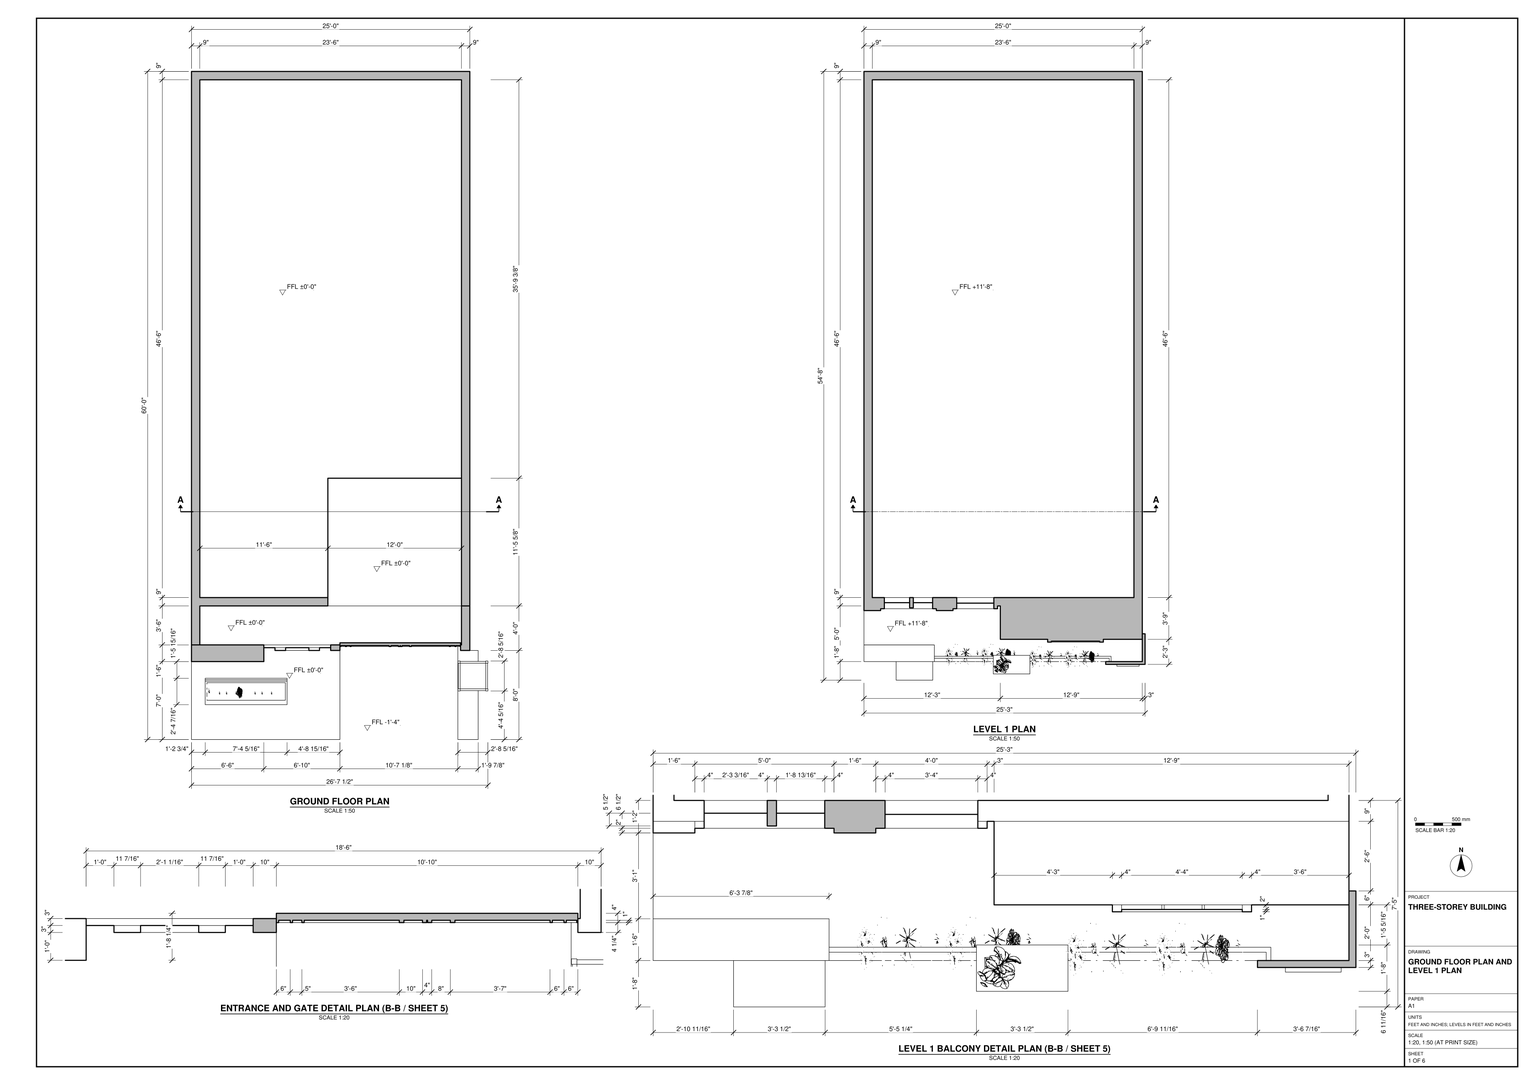
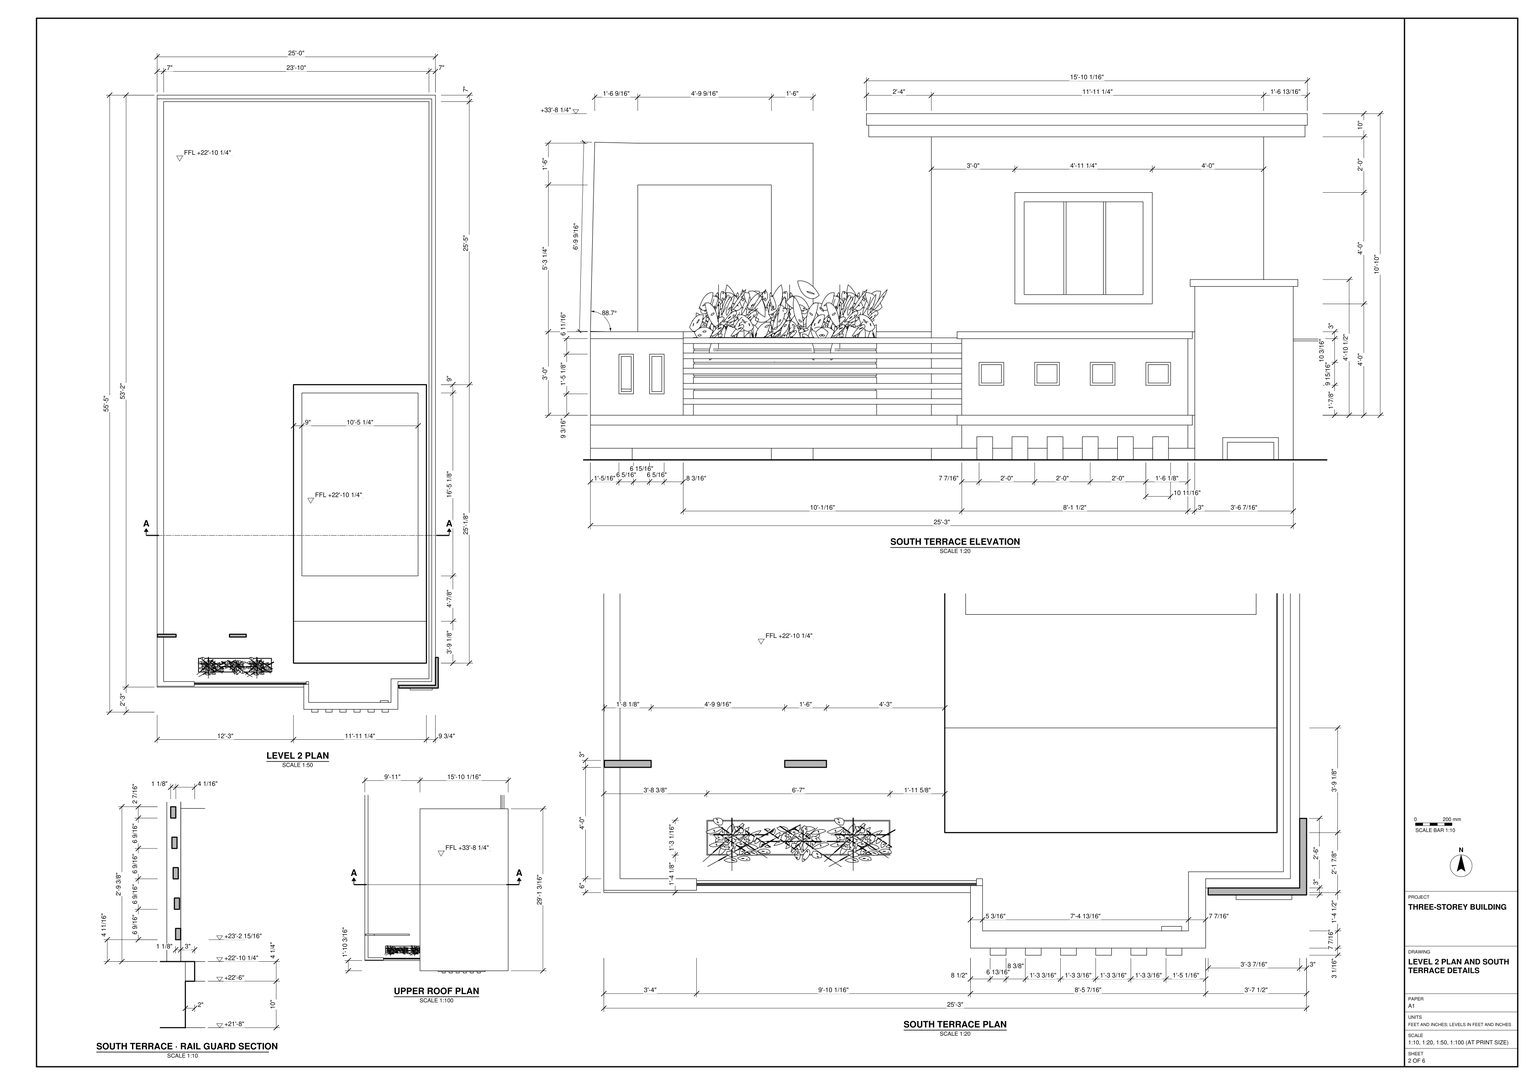
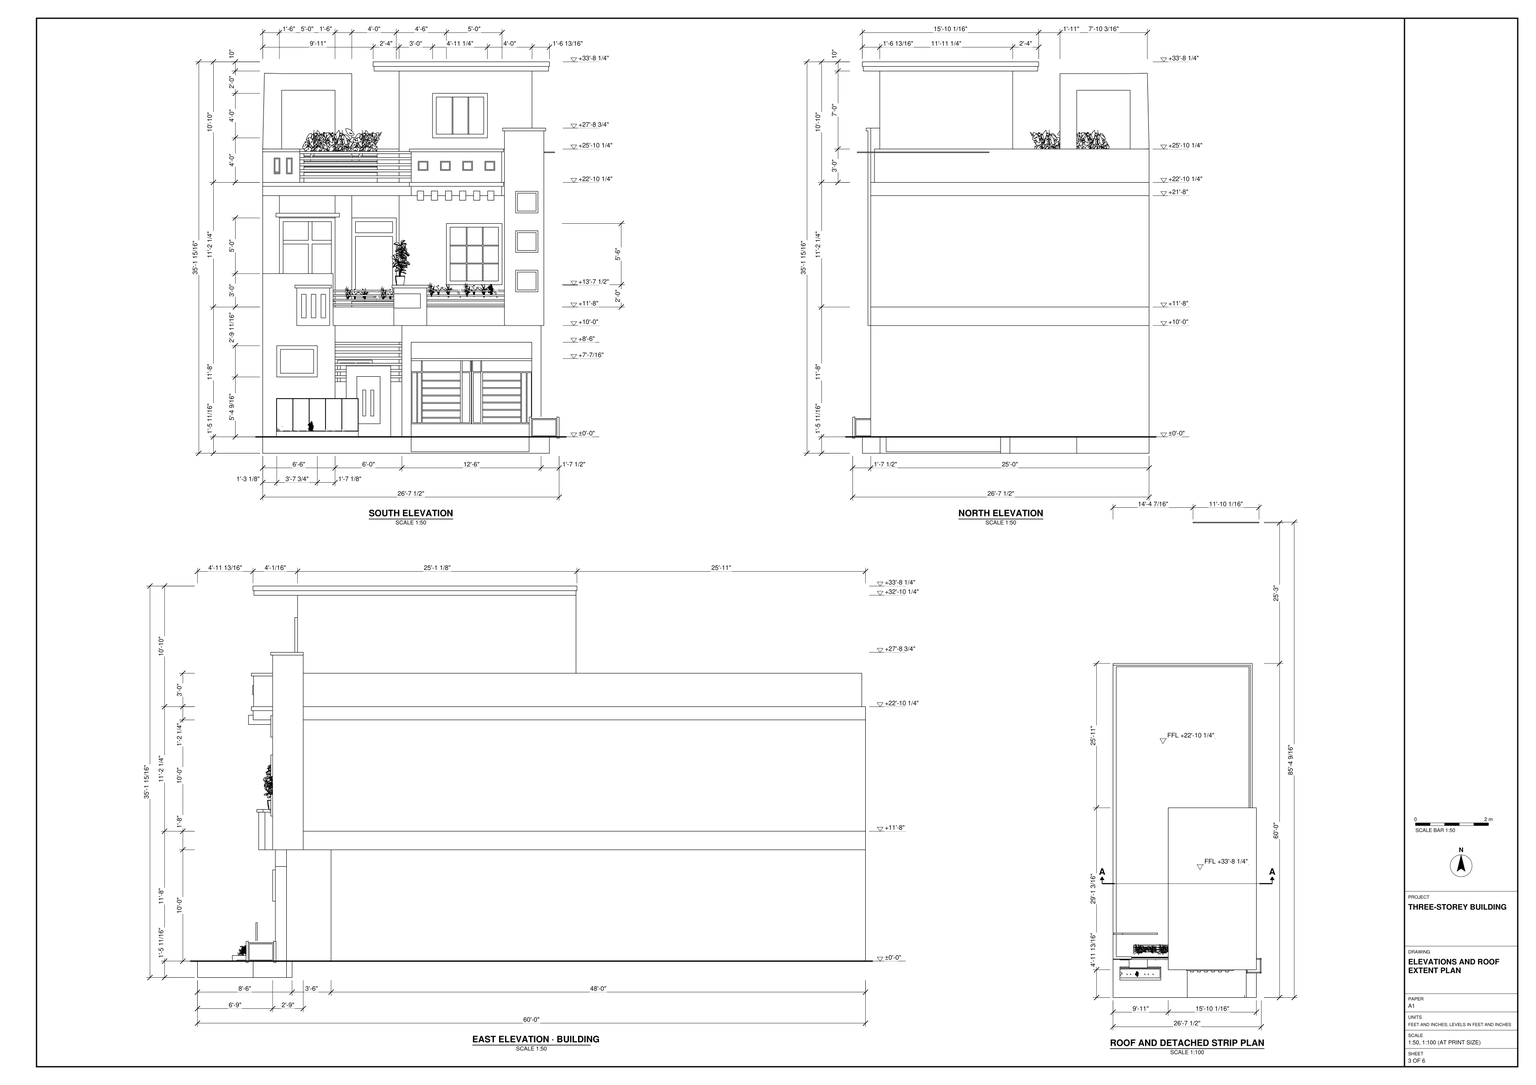
Build the three-storey building in SketchUp from task_files/diagram_01.pdf. Work in feet and inches. The complete model is 26'-7 1/2" wide, 85'-4 9/16" deep and 35'-1 15/16" high. Use finished floor levels of ±0'-0", +11'-8" and +22'-10 1/4". The overall depth includes the detached strip; position it from the roof and detached strip plan rather than extending the building to fill that depth.

Lay out the slabs and walls from the floor plans, using the 9" main perimeter walls on the lower floors and the 7" terrace perimeter walls where dimensioned. Keep the rear and long side elevations plain as drawn. On the south front, model the change in ground level, pedestrian entrance, wider slatted gate and projecting balcony. Set the balcony door and divided windows behind the guard, and carry the tall panelled feature up the right edge of the facade. At terrace level, distinguish the open frame from the roofed enclosure. Follow the terrace details for the parapet openings, horizontal rails and planting positions.

Decor and loose items, including plants, may be any suitable library components, for example from 3D Warehouse. Keep shell elements such as walls, slabs and roofs, and each furniture or joinery piece shown, in separate groups or components. Use components for repeated parts. Save one SketchUp model as output_files/three_storey_building_south_balcony_and_roof_terrace.skp.

# SketchUp Ruby script. Lengths in inches.
U = 1.inch
M = Sketchup.active_model
def pt(a) = Geom::Point3d.new(a.map { |v| v * U })
def face(e, loops, mat)
  f = e.add_face(loops[0].map { |a| pt(a) })
  loops[1..].each { |l| e.add_face(l.map { |a| pt(a) }).erase! }
  f.material = f.back_material = mat if mat
  f
end
# faces: each face lists its corners as indices into pts; further lists are holes
def faces(e, pts, list, mat = nil) = list.each { |f| face(e, (f[0].is_a?(Array) ? f : [f]).map { |l| l.map { |i| pts[i] } }, mat) }
# xy, xz, yz: faces in a plane at the given z, y or x. An outline is a flat list of corners, or four numbers for a rectangle; further outlines are holes
def ring(l) = l.size == 4 ? [[l[0], l[1]], [l[2], l[1]], [l[2], l[3]], [l[0], l[3]]] : l.each_slice(2).to_a
def flat(e, list, mat, &to3) = list.each { |f| face(e, (f[0].is_a?(Array) ? f : [f]).map { |l| ring(l).map { |u, v| to3.(u, v) } }, mat) }
def xy(e, z, list, mat = nil) = flat(e, list, mat) { |x, y| [x, y, z] }
def xz(e, y, list, mat = nil) = flat(e, list, mat) { |x, z| [x, y, z] }
def yz(e, x, list, mat = nil) = flat(e, list, mat) { |y, z| [x, y, z] }
def lines(e, pts, list) = list.each { |a, b| e.add_line(pt(pts[a]), pt(pts[b])) }
# prism: a flat outline (further loops are holes) pulled along v
def prism(e, loops, v, mat = nil)
  f = face(e, loops, mat); d = Geom::Vector3d.new(v.map { |x| x * U })
  f.pushpull(f.normal.samedirection?(d) ? d.length : -d.length)
end
def box(e, o, s, mat = nil) = prism(e, [[o, [o[0] + s[0], o[1], o[2]], [o[0] + s[0], o[1] + s[1], o[2]], [o[0], o[1] + s[1], o[2]]]], [0, 0, s[2]], mat)
def at(x, y, z, deg = 0) = Geom::Transformation.translation(pt([x, y, z])) * Geom::Transformation.rotation(ORIGIN, Z_AXIS, deg.degrees)
def axes(o, x, y, z) = Geom::Transformation.new([*x, 0, *y, 0, *z, 0, *pt(o).to_a, 1])
def part(name) = M.definitions.add(name)
# library, detail: a bought-in or finely detailed component or shape, given as its bounding box
def library(name, o, s) = part(name).tap { |d| box(d.entities, o, s) }
def detail(e, o, s) = box(e.add_group.entities, o, s)
def put(e, d, t, mat = nil) = e.add_instance(d, t).tap { |i| i.material = mat if mat }
def group(e, t, mat = nil) = e.add_group.tap { |g| g.transformation = t; g.material = mat if mat }.entities
root = M.entities
M.materials.add("Brick_05_1K1").color = [143, 147, 94]
M.materials.add("Brick_05_1K2").color = [195, 185, 161]
M.materials.add("Brick_21_1K").color = [96, 58, 28]
M.materials.add("D01_Frost_White").color = [255, 242, 206]
M.materials.add("Glass_Basic_01").color = [161, 173, 186]
M.materials["Glass_Basic_01"].alpha = 0.25
M.materials.add("Glass_Mirror_01").color = [158, 180, 198]
M.materials.add("Glass_Mirror_1").color = [163, 154, 154]
M.materials.add("Glass_Mirror_2").color = [147, 150, 185]
M.materials.add("Marble_01_1K").color = [230, 221, 211]
M.materials.add("Material__1").color = [95, 70, 46]
M.materials.add("Plywood_01_1K").color = [125, 96, 64]
M.materials.add("Tile_Exterior_07_1K").color = [112, 111, 107]
M.materials.add("Wood_Veneer_15_1K").color = [103, 69, 45]
M.materials.add("[Color M00]").color = [255, 255, 255]
M.materials.add("[Translucent Glass Gray]").color = [128, 128, 128]
M.materials["[Translucent Glass Gray]"].alpha = 0.29
c1 = part("Roof terrace")
xy(c1.entities,-5,[[166.59,-89,173.41,-40.3125],[181.75,-89,188.57,-40.3125],[196.92,-89,203.73,-40.3125],[212.08,-89,218.9,-40.3125],[227.25,-89,234.0625,-40.3125],
  [242.41,-89,249.23,-40.3125]],"Wood_Veneer_15_1K")
xy(c1.entities,0,[[160.08,-84,160.08,-60,0,-60,0,576,300,576,300,-60,257.58,-60,257.58,-84,249.23,-84,249.23,-40.3125,242.41,-40.3125,242.41,-84,234.0625,-84,234.0625,-40.3125,227.25,-40.3125,227.25,-84,218.9,-84,218.9,-40.3125,212.08,-40.3125,212.08,-84,203.73,-84,203.73,-40.3125,196.92,-40.3125,196.92,-84,188.57,-84,188.57,-40.3125,181.75,-40.3125,181.75,-84,173.41,-84,173.41,-40.3125,166.59,-40.3125,166.59,-84],[166.59,-84,173.41,-40.3125],[181.75,-84,188.57,-40.3125],[196.92,-84,203.73,-40.3125],[212.08,-84,218.9,-40.3125],
  [227.25,-84,234.0625,-40.3125],[242.41,-84,249.23,-40.3125]])
xy(c1.entities,5,[[166.59,-89,173.41,-84],[181.75,-89,188.57,-84],[196.92,-89,203.73,-84],[212.08,-89,218.9,-84],[227.25,-89,234.0625,-84],
  [242.41,-89,249.23,-84]],"Wood_Veneer_15_1K")
xy(c1.entities,10,[[158.08,-85.91,158.08,-84,257.58,-84,257.58,-60,259.5,-60,259.5,-85.91],[158.08,-84,160.08,-65],[158.08,-65,160.08,-62],[0,-62,160.08,-60]])
xy(c1.entities,14.24,[[[158.08,-85.91,259.5,-85.91,259.5,-60,300,-60,300,576,0,576,0,572,296,572,296,-56,257.58,-56,257.58,-83.5,160.08,-83.5,160.08,-59,163.28,-59,163.28,-78.5,252.08,-78.5,252.08,-53,293,-53,293,569,7,569,7,-56,40,-56,40,-59,0,-59,0,-62,158.08,-62],[147,-36.12,290.25,264],[78,-8,96,-5],[18,-8,20.41,-5]],[160.08,-83.5,257.58,-83.5,257.58,-56,296,-56,296,572,0,572,0,-59,40,-59,40,-56,7,-56,7,569,293,569,293,-53,252.08,-53,252.08,-78.5,163.28,-78.5,163.28,-59,160.08,-59],[18,-8,20.41,-5],[78,-8,96,-5],[156,57.91,281.25,255]])
xy(c1.entities,23.4375,[[12.29,-60,18.58,-59],[25.5,-60,31.79,-59]])
xy(c1.entities,24.4375,[[13.29,-60,17.58,-56],[26.5,-60,30.79,-56]])
xy(c1.entities,27.13,[[167.54,-84.5,178.21,-83.5],[191.52,-84.5,202.1875,-83.5],[215.49,-84.5,226.16,-83.5]])
xy(c1.entities,28.13,[[168.54,-84.5,177.21,-78.5],[192.52,-84.5,201.1875,-78.9375],[216.49,-84.5,225.16,-78.5],[240.47,-83.5,249.14,-78.5],[192.52,-78.9375,201.1875,-78.5],
  [240.47,-78.5,249.14,-76.55]])
xy(c1.entities,36.05,[[168.54,-84.5,177.21,-78.5],[192.52,-84.5,201.1875,-78.9375],[216.49,-84.5,225.16,-78.5],[240.47,-83.5,249.14,-76.55],[192.52,-78.9375,201.1875,-78.5]])
xy(c1.entities,37.05,[[167.54,-84.5,178.21,-83.5],[191.52,-84.5,202.1875,-83.5],[215.49,-84.5,226.16,-83.5]])
xy(c1.entities,39.58,[[13.29,-60,17.58,-56],[26.5,-60,30.79,-56]])
xy(c1.entities,40.58,[[12.29,-60,18.58,-59],[25.5,-60,31.79,-59]])
xy(c1.entities,46.29,[[172.45,879,314.53,880.56]])
xy(c1.entities,47.08,[[172.45,879,314.53,880.56]])
xy(c1.entities,47.24,[[158.08,-85.91,160.08,-59],[160.08,-85.91,160.08,-83.5,257.58,-83.5,257.58,-56,259.5,-56,259.5,-85.91],[0,-61,40,-59]])
xy(c1.entities,50.24,[[158.08,-85.91,259.5,-85.91,259.5,-56,296,-56,296,572,0,572,0,-61,40,-61,40,-56,7,-56,7,569,293,569,293,-53,252.08,-53,252.08,-78.5,163.28,-78.5,163.28,-59,158.08,-59]])
xy(c1.entities,62.24,[[183,-39.12,242.25,-36.12]])
xy(c1.entities,66.24,[[187,-39.12,204.08,-36.12],[204.08,-39.12,205.08,-38.12],[205.08,-39.12,221.17,-36.12],[221.17,-39.12,222.17,-36.12],[222.17,-39.12,238.25,-36.12]])
xy(c1.entities,106.24,[[187,-39.12,204.08,-36.12],[204.08,-39.12,205.08,-38.12],[205.08,-39.12,221.17,-36.12],[221.17,-39.12,222.17,-36.12],[222.17,-39.12,238.25,-36.12]])
xy(c1.entities,110.24,[[183,-39.12,242.25,-36.12]])
xy(c1.entities,113.51,[[20.41,-8,78,-5]],"Plywood_01_1K")
xy(c1.entities,131.51,[[20.41,-8,96,-5]])
xy(c1.entities,134.24,[[147,-36.12,290.25,264]])
xy(c1.entities,139.24,[[119.99,-83.16,308.08,264]])
xz(c1.entities,-89,[[166.59,-5,173.41,5],[181.75,-5,188.57,5],[196.92,-5,203.73,5],[212.08,-5,218.9,5],[227.25,-5,234.0625,5],
  [242.41,-5,249.23,5]],"Wood_Veneer_15_1K")
xz(c1.entities,-85.91,[[158.08,10,259.5,14.24],[158.08,47.24,259.5,50.24]])
xz(c1.entities,-84.5,[[[167.54,27.13,178.21,37.05],[168.54,28.13,177.21,36.05]],[[191.52,27.13,202.1875,37.05],[192.52,28.13,201.1875,36.05]],[[215.49,27.13,226.16,37.05],[216.49,28.13,225.16,36.05]]])
xz(c1.entities,-84,[[160.08,0,166.59,0,166.59,5,173.41,5,173.41,0,181.75,0,181.75,5,188.57,5,188.57,0,196.92,0,196.92,5,203.73,5,203.73,0,212.08,0,212.08,5,218.9,5,218.9,0,227.25,0,227.25,5,234.0625,5,234.0625,0,242.41,0,242.41,5,249.23,5,249.23,0,257.58,0,257.58,10,160.08,10],[166.59,0,173.41,5],[181.75,0,188.57,5],[196.92,0,203.73,5],[212.08,0,218.9,5],
  [227.25,0,234.0625,5],[242.41,0,249.23,5]])
xz(c1.entities,-83.5,[[[160.08,14.24,257.58,47.24],[167.54,27.13,178.21,37.05],[191.52,27.13,202.1875,37.05],[215.49,27.13,226.16,37.05],[239.47,27.13,250.14,37.05]],[[239.47,27.13,250.14,37.05],[240.47,28.13,249.14,36.05]]])
xz(c1.entities,-78.5,[[163.28,14.24,168.54,36.05],[168.54,14.24,249.28,28.13],[249.28,14.24,252.08,36.49],[177.21,28.13,192.52,36.05],[201.1875,28.13,216.49,36.05],
  [163.28,36.05,233.07,50.24],[233.07,36.49,252.08,50.24]])
xz(c1.entities,-62,[[0,10,158.08,14.24]])
xz(c1.entities,-61,[[0,47.24,40,50.24]])
xz(c1.entities,-60,[[0,0,160.08,10],[257.58,0,270,0,270,14.24,259.5,14.24,259.5,10,257.58,10],[270,0,300,14.24],[[12.29,23.4375,18.58,40.58],[13.29,24.4375,17.58,39.58]],[[25.5,23.4375,31.79,40.58],[26.5,24.4375,30.79,39.58]]])
xz(c1.entities,-59,[[[0,14.24,40,47.24],[12.29,23.4375,18.58,40.58],[25.5,23.4375,31.79,40.58]],[160.08,14.24,163.28,47.24],[158.08,47.24,163.28,50.24]])
xz(c1.entities,-56,[[[7,14.24,40,50.24],[26.5,24.4375,30.79,39.58],[13.29,24.4375,17.58,39.58]],[257.58,14.24,296,14.24,296,50.24,259.5,50.24,259.5,47.24,257.58,47.24]])
xz(c1.entities,-53,[[252.08,14.24,270,50.24],[270,14.24,293,50.24]])
xz(c1.entities,-40.3125,[[227.25,-5,234.0625,0],[242.41,-5,249.23,0]])
xz(c1.entities,-40.3125,[[166.59,-5,173.41,0],[181.75,-5,188.57,0],[196.92,-5,203.73,0],[212.08,-5,218.9,0]],"Wood_Veneer_15_1K")
xz(c1.entities,-39.12,[[[183,62.24,242.25,110.24],[187,66.24,238.25,106.24]]])
xz(c1.entities,-38.12,[[204.08,66.24,205.08,106.24]])
xz(c1.entities,-36.12,[[221.17,66.24,222.17,106.24]])
xz(c1.entities,-36.12,[[[147,14.24,290.25,134.24],[183,62.24,242.25,110.24]]],"Brick_05_1K1")
xz(c1.entities,-36.12,[[187,66.24,204.08,106.24],[205.08,66.24,221.17,106.24],[222.17,66.24,238.25,106.24]],"Glass_Basic_01")
xz(c1.entities,-8,[[18,14.24,20.41,14.24,20.41,113.51,78,113.51,78,14.24,96,14.24,96,131.51,20.41,131.51,1.86,131.93,0,50.4,7,50.24,6.44,25.74,18,25.48]],"Plywood_01_1K")
xz(c1.entities,-5,[[18,14.24,18,25.48,6.44,25.74,7,50.24,0,50.4,1.86,131.93,20.41,131.51,96,131.51,96,14.24,78,14.24,78,113.51,20.41,113.51,20.41,14.24]],"Plywood_01_1K")
xz(c1.entities,264,[[147,14.24,290.25,134.24]])
xz(c1.entities,569,[[7,14.24,293,50.24]])
xz(c1.entities,572,[[0,14.24,296,50.24]])
xz(c1.entities,576,[[0,0,300,14.24]])
xz(c1.entities,879,[[172.45,46.29,314.53,47.08]])
xz(c1.entities,880.56,[[172.45,46.29,314.53,47.08]])
yz(c1.entities,0,[[-60,0,-60,10,-62,10,-62,14.24,576,14.24,576,0],[-59,14.24,-59,47.24,-61,47.24,-61,50.24,572,50.24,572,14.24]])
yz(c1.entities,7,[[-56,14.24,569,50.24]])
yz(c1.entities,12.29,[[-60,23.4375,-59,40.58]])
yz(c1.entities,13.29,[[-60,24.4375,-56,39.58]])
yz(c1.entities,17.58,[[-60,24.4375,-56,39.58]])
yz(c1.entities,18,[[-8,14.24,-5,25.48]])
yz(c1.entities,18.58,[[-60,23.4375,-59,40.58]])
yz(c1.entities,20.41,[[-8,14.24,-5,113.51]],"Plywood_01_1K")
yz(c1.entities,25.5,[[-60,23.4375,-59,40.58]])
yz(c1.entities,26.5,[[-60,24.4375,-56,39.58]])
yz(c1.entities,30.79,[[-60,24.4375,-56,39.58]])
yz(c1.entities,31.79,[[-60,23.4375,-59,40.58]])
yz(c1.entities,40,[[[-59,14.24,-56,14.24,-56,50.24,-61,50.24,-61,47.24,-59,47.24],[-57.94,45.71,-56.84,47.61]]])
yz(c1.entities,78,[[-8,14.24,-5,113.51]],"Plywood_01_1K")
yz(c1.entities,96,[[-8,14.24,-5,23.51],[-8,23.51,-5,107.51],[-8,107.51,-5,131.51]],"Plywood_01_1K")
yz(c1.entities,147,[[-36.12,14.24,264,134.24]])
yz(c1.entities,158.08,[[-85.91,10,-62,14.24],[-85.91,47.24,-59,50.24]])
yz(c1.entities,160.08,[[-84,0,-60,10],[-83.5,14.24,-59,47.24]])
yz(c1.entities,163.28,[[-78.5,14.24,-78.25,50.24],[-78.25,14.24,-59,50.24]])
yz(c1.entities,166.59,[[-89,-5,-89,5,-84,5,-84,0,-40.3125,0,-40.3125,-5]],"Wood_Veneer_15_1K")
yz(c1.entities,167.54,[[-84.5,27.13,-83.5,37.05]])
yz(c1.entities,168.54,[[-84.5,28.13,-78.5,36.05]])
yz(c1.entities,173.41,[[-89,-5,-40.3125,-5,-40.3125,0,-84,0,-84,5,-89,5]],"Wood_Veneer_15_1K")
yz(c1.entities,177.21,[[-84.5,28.13,-78.5,36.05]])
yz(c1.entities,178.21,[[-84.5,27.13,-83.5,37.05]])
yz(c1.entities,181.75,[[-89,-5,-89,5,-84,5,-84,0,-40.3125,0,-40.3125,-5]],"Wood_Veneer_15_1K")
yz(c1.entities,183,[[-39.12,62.24,-36.12,110.24]])
yz(c1.entities,187,[[-39.12,66.24,-36.12,106.24]])
yz(c1.entities,188.57,[[-89,-5,-40.3125,-5,-40.3125,0,-84,0,-84,5,-89,5]],"Wood_Veneer_15_1K")
yz(c1.entities,191.52,[[-84.5,27.13,-83.5,37.05]])
yz(c1.entities,192.52,[[-84.5,28.13,-78.9375,36.05],[-78.9375,28.13,-78.5,36.05]])
yz(c1.entities,196.92,[[-89,-5,-89,5,-84,5,-84,0,-40.3125,0,-40.3125,-5]],"Wood_Veneer_15_1K")
yz(c1.entities,201.1875,[[-84.5,28.13,-78.9375,36.05],[-78.9375,28.13,-78.5,36.05]])
yz(c1.entities,202.1875,[[-84.5,27.13,-83.5,37.05]])
yz(c1.entities,203.73,[[-89,-5,-40.3125,-5,-40.3125,0,-84,0,-84,5,-89,5]],"Wood_Veneer_15_1K")
yz(c1.entities,204.08,[[-38.12,66.24,-36.12,106.24]])
yz(c1.entities,205.08,[[-38.12,66.24,-36.12,106.24]])
yz(c1.entities,212.08,[[-89,-5,-89,5,-84,5,-84,0,-40.3125,0,-40.3125,-5]],"Wood_Veneer_15_1K")
yz(c1.entities,215.49,[[-84.5,27.13,-83.5,37.05]])
yz(c1.entities,216.49,[[-84.5,28.13,-78.5,36.05]])
yz(c1.entities,218.9,[[-89,-5,-40.3125,-5,-40.3125,0,-84,0,-84,5,-89,5]],"Wood_Veneer_15_1K")
yz(c1.entities,225.16,[[-84.5,28.13,-78.5,36.05]])
yz(c1.entities,226.16,[[-84.5,27.13,-83.5,37.05]])
yz(c1.entities,227.25,[[-89,-5,-89,5,-84,5,-84,0,-40.3125,0,-40.3125,-5]],"Wood_Veneer_15_1K")
yz(c1.entities,234.0625,[[-89,-5,-40.3125,-5,-40.3125,0,-84,0,-84,5,-89,5]],"Wood_Veneer_15_1K")
yz(c1.entities,238.25,[[-39.12,66.24,-36.12,106.24]])
yz(c1.entities,240.47,[[-83.5,28.13,-76.55,36.05]])
yz(c1.entities,242.25,[[-39.12,62.24,-36.12,110.24]])
yz(c1.entities,242.41,[[-89,-5,-89,5,-84,5,-84,0,-40.3125,0,-40.3125,-5]],"Wood_Veneer_15_1K")
yz(c1.entities,249.14,[[-83.5,28.13,-76.55,36.05]])
yz(c1.entities,249.23,[[-89,-5,-40.3125,-5,-40.3125,0,-84,0,-84,5,-89,5]],"Wood_Veneer_15_1K")
yz(c1.entities,252.08,[[-78.5,14.24,-53,50.24]])
yz(c1.entities,257.58,[[-84,0,-60,10],[-83.5,14.24,-56,47.24]])
yz(c1.entities,259.5,[[-85.91,10,-60,14.24],[-85.91,47.24,-56,50.24]])
yz(c1.entities,290.25,[[-36.12,14.24,264,134.24]])
yz(c1.entities,293,[[-53,14.24,569,50.24]])
yz(c1.entities,296,[[-56,14.24,572,50.24]])
yz(c1.entities,300,[[-60,0,576,14.24]])
p = [[18,-5,25.48],[18,-8,25.48],[6.44,-8,25.74],[6.44,-5,25.74],[7,-8,50.24],[7,-5,50.24],
  [0,-8,50.4],[0,-5,50.4],[1.86,-5,131.93],[1.86,-8,131.93],[20.41,-8,131.51],[20.41,-5,131.51],
  [156,57.91,14.24],[156,57.91,134.24],[281.25,57.91,14.24],[281.25,57.91,134.24],[156,255,14.24],[156,255,134.24],
  [281.25,255,14.24],[281.25,255,134.24],[18,-5,0],[18,-5,14.24],[96,-5,0],[96,-5,14.24]]
faces(c1.entities,p,[[0,1,2,3],[2,4,5,3],[5,4,6,7],[10,11,8,9]])
faces(c1.entities,p,[[8,7,6,9]],"Plywood_01_1K")
lines(c1.entities,p,[[12,13],[14,15],[16,17],[18,19],[20,21],[22,23]])
g1 = group(c1.entities,at(40,-58.74,25.51))
xy(g1,0,[[0,0,123.28,1.1]])
xy(g1,2.43,[[0,0,123.28,1.1]])
xz(g1,0,[[0,0,123.28,2.43]])
xz(g1,1.1,[[0,0,123.28,2.43]])
yz(g1,123.28,[[0,0,1.1,2.43]])
g2 = group(c1.entities,at(40,-59,18.95))
xy(g2,0,[[0,0,123.28,1.1]])
xy(g2,2.43,[[0,0,123.28,1.1]])
xz(g2,0,[[0,0,123.28,2.43]])
xz(g2,1.1,[[0,0,123.28,2.43]])
yz(g2,123.28,[[0,0,1.1,2.43]])
g3 = group(c1.entities,at(40,-58.21,38.62))
xy(g3,0,[[0,0,123.28,1.1]])
xy(g3,2.43,[[0,0,123.28,1.1]])
xz(g3,0,[[0,0,123.28,2.43]])
xz(g3,1.1,[[0,0,123.28,2.43]])
yz(g3,123.28,[[0,0,1.1,2.43]])
g4 = group(c1.entities,at(40,-57.94,45.17))
xy(g4,0,[[0,0,123.28,1.1]])
xy(g4,2.43,[[0,0,123.28,1.1]])
xz(g4,0,[[0,0,123.28,2.43]])
xz(g4,1.1,[[0,0,123.28,2.43]])
yz(g4,123.28,[[0,0,1.1,2.43]])
g5 = group(c1.entities,at(40,-58.47,32.0625))
xy(g5,0,[[0,0,123.28,1.1]])
xy(g5,2.43,[[0,0,123.28,1.1]])
xz(g5,0,[[0,0,123.28,2.43]])
xz(g5,1.1,[[0,0,123.28,2.43]])
yz(g5,123.28,[[0,0,1.1,2.43]])
g6 = group(c1.entities,at(119.99,-83.16,134.24))
xy(g6,0,[[0,0,188.09,347.16]])
xy(g6,5,[[-1,-1,189.09,0],[-1,0,0,348.16],[0,0,188.09,347.16],[188.09,0,189.09,348.16],[0,347.16,188.09,348.16]])
xy(g6,10,[[-1,-1,189.09,348.16]])
xz(g6,-1,[[-1,5,189.09,10]],"Brick_21_1K")
xz(g6,0,[[0,0,188.09,5]])
xz(g6,347.16,[[0,0,188.09,5]])
xz(g6,348.16,[[-1,5,189.09,10]],"Brick_21_1K")
yz(g6,-1,[[-1,5,348.16,10]],"Brick_21_1K")
yz(g6,0,[[0,0,347.16,5]])
yz(g6,188.09,[[0,0,347.16,5]])
yz(g6,189.09,[[-1,5,348.16,10]],"Brick_21_1K")
c2 = library("Planted timber trough",[0,0,0],[56.02,15.3,25.28])
c3 = library("Areca palm plant",[0,0,0],[49.1,36.6,54.46])
c4 = part("W1")
xy(c4.entities,15,[[0,0,2,198]])
xy(c4.entities,102.0625,[[0,0,2,198]],"[Color M00]")
xz(c4.entities,0,[[0,15,2,102.0625]],"[Color M00]")
xz(c4.entities,198,[[0,15,2,102.0625]])
yz(c4.entities,0,[[0.84,16,39.43,101.0625],[40.28,16,78.87,101.0625],[79.71,16,118.3,101.0625],[119.14,16,157.73,101.0625],[158.58,16,197.16,101.0625]])
yz(c4.entities,0,[[[0,15,198,102.0625],[0.84,16,197.16,101.0625]],[39.43,16,40.28,101.0625],[78.87,16,79.71,101.0625],[118.3,16,119.14,101.0625],[157.73,16,158.58,101.0625]],"[Color M00]")
yz(c4.entities,2,[[0.84,16,39.43,101.0625],[40.28,16,78.87,101.0625],[79.71,16,118.3,101.0625],[119.14,16,157.73,101.0625],[158.58,16,197.16,101.0625]])
yz(c4.entities,2,[[[0,15,198,102.0625],[0.84,16,197.16,101.0625]],[39.43,16,40.28,101.0625],[78.87,16,79.71,101.0625],[118.3,16,119.14,101.0625],[157.73,16,158.58,101.0625]],"[Color M00]")
c5 = library("Group\#74",[-84.69,-90.07,-0.36],[176.51,175.13,171.4])
c6 = library("Group20\#1",[-20.81,-17.08,3.79],[39.86,39.43,37.51])
c7 = library("Group\#130",[-7.34,-1.2,0],[38.67,35.81,49.04])
c8 = library("Group38\#2",[14.01,28.44,-23.43],[18.58,18.32,38.89])
c9 = part("PLANTS (1)")
put(c9.entities,c3,axes([90.35,-3.44,359.07],[0.45017,-0.56191,0],[0.66137,0.52986,0],[0,0,0.72]))
put(c9.entities,c3,axes([90.35,-105.25,359.07],[0.45017,-0.56191,0],[0.66137,0.52986,0],[0,0,0.72]))
put(c9.entities,c4,axes([76.68,11.43,-0.0625],[1,0,0],[0,1.18586,0],[0,0,1]),"[Translucent Glass Gray]")
put(c9.entities,c3,axes([87.03,-243.25,369.41],[0.45017,-0.56191,0],[0.66137,0.52986,0],[0,0,0.72]))
put(c9.entities,c3,axes([87.03,-345.06,369.41],[0.45017,-0.56191,0],[0.66137,0.52986,0],[0,0,0.72]))
put(c9.entities,c5,axes([59.61,184.54,5.99],[-0.04961,-0.08593,0],[0.08593,-0.04961,0],[0,0,0.10522]))
put(c9.entities,c5,axes([59.61,204.61,5.99],[-0.04961,-0.08593,0],[0.08593,-0.04961,0],[0,0,0.10522]))
put(c9.entities,c5,axes([59.61,157.29,5.99],[-0.04961,-0.08593,0],[0.08593,-0.04961,0],[0,0,0.10522]))
put(c9.entities,c6,axes([115.52,-81.875,357.77],[0,0.85,0],[-0.85,0,0],[0,0,0.85]))
put(c9.entities,c7,axes([121.49,-71.94,360.99],[0,0.79,0],[-0.79,0,0],[0,0,0.79]))
put(c9.entities,c8,axes([92.44,-163.01,381.16],[0.8848,0,0],[0,0.94674,0],[0,0,0.85826]))
put(c9.entities,c5,axes([59.61,55.48,5.99],[-0.04961,-0.08593,0],[0.08593,-0.04961,0],[0,0,0.10522]))
put(c9.entities,c5,axes([59.61,82.73,5.99],[-0.04961,-0.08593,0],[0.08593,-0.04961,0],[0,0,0.10522]))
put(c9.entities,c5,axes([113.74,-40.62,359.07],[-0.08133,-0.14087,0],[0.14087,-0.08133,0],[0,0,0.1725]))
put(c9.entities,c5,axes([59.61,102.79,5.99],[-0.04961,-0.08593,0],[0.08593,-0.04961,0],[0,0,0.10522]))
put(c9.entities,c5,axes([113.74,-146.06,359.07],[-0.08133,-0.14087,0],[0.14087,-0.08133,0],[0,0,0.1725]))
put(c9.entities,c5,axes([61.875,234.47,6.01],[-0.08133,-0.14087,0],[0.14087,-0.08133,0],[0,0,0.1725]))
put(c9.entities,c7,axes([121.49,29.87,360.99],[0,0.79,0],[-0.79,0,0],[0,0,0.79]))
put(c9.entities,c6,axes([115.52,19.9375,357.77],[0,0.85,0],[-0.85,0,0],[0,0,0.85]))
put(c9.entities,c8,axes([40.58,112.08,28.11],[0.8848,0,0],[0,0.94674,0],[0,0,0.85826]))
g7 = group(c9.entities,at(44.68,11.43,-0.0625))
xy(g7,0,[[0,0,6,234.8],[30,0,36,234.8]])
xy(g7,3,[[6,0,30,234.8]])
xy(g7,7,[[6,5,30,229.8]],"Material__1")
xy(g7,15,[[[0,0,36,234.8],[6,5,30,229.8]]])
xz(g7,0,[[0,0,6,0,6,3,30,3,30,0,36,0,36,15,0,15]])
xz(g7,5,[[6,7,30,15]])
xz(g7,229.8,[[6,7,30,15]])
xz(g7,234.8,[[0,0,0,15,36,15,36,0,30,0,30,3,6,3,6,0]])
yz(g7,0,[[0,0,234.8,15]])
yz(g7,6,[[0,0,234.8,3],[5,7,229.8,15]])
yz(g7,30,[[0,0,234.8,3],[5,7,229.8,15]])
yz(g7,36,[[0,0,234.8,15]])
put(c9.entities,c5,axes([110.42,-385.86,369.41],[-0.08133,-0.14087,0],[0.14087,-0.08133,0],[0,0,0.1725]))
put(c9.entities,c7,axes([118.16,-311.75,371.33],[0,0.79,0],[-0.79,0,0],[0,0,0.79]))
put(c9.entities,c7,axes([118.16,-209.93,371.33],[0,0.79,0],[-0.79,0,0],[0,0,0.79]))
put(c9.entities,c8,axes([89.12,-402.81,391.5],[0.8848,0,0],[0,0.94674,0],[0,0,0.85826]))
put(c9.entities,c6,axes([112.19,-321.68,368.1],[0,0.85,0],[-0.85,0,0],[0,0,0.85]))
put(c9.entities,c5,axes([110.42,-280.42,369.41],[-0.08133,-0.14087,0],[0.14087,-0.08133,0],[0,0,0.1725]))
put(c9.entities,c6,axes([112.19,-219.87,368.1],[0,0.85,0],[-0.85,0,0],[0,0,0.85]))
c10 = library("Group_2",[-1.28,-0.39,0],[21.22,20.51,48.44])
c11 = library("Potted tree",[0,0,-1.57],[32.28,32.28,23.42])
c12 = library("Group\#10",[0,0,0],[130,4,72])
c13 = part("Group\#15")
box(c13.entities,[0,0,0],[2.74,2.54,12])
c14 = library("Group\#17",[-2,0,0],[39.47,43.48,20])
box(root,[73.57,87.58,156.46],[67.82,2.15,1.65],"D01_Frost_White")
box(root,[75.8,87.58,146.64],[65.59,2.15,1.66],"D01_Frost_White")
box(root,[75.8,87.58,141.74],[65.59,2.15,1.65],"D01_Frost_White")
xy(root,-17.6875,[[[0,0,0,84,78,84,78,102,150,102,150,96,160,96,160,102,290,102,290,96,308.98,96,308.98,0],[90,96,138,99]]],"D01_Frost_White")
xy(root,-16.02,[[160,0,283.35,102]],"D01_Frost_White")
xy(root,0,[[[0,0,160,0,160,96,150,96,150,102,78,102,78,84,0,84],[90,96,138,99]],[287.1,0,308.98,0,308.98,96,290,96,290,102,287.1,102]],"Brick_05_1K2")
xy(root,0,[[0,84,78,102],[90,96,138,99],[150,96,160,102],[290,96,300,96,300,144,291,144,291,102,290,102],[0,102,9,144],
  [9,102,291,144]],"D01_Frost_White")
xy(root,14.19,[[101.47,96,126.53,99]],"D01_Frost_White")
xy(root,64.59,[[15.14,81,58.88,84]],"D01_Frost_White")
xy(root,65.06,[[101.47,96,126.53,99]],"D01_Frost_White")
xy(root,68.59,[[19.14,81,54.88,93],[19.14,93,54.88,102]],"D01_Frost_White")
xy(root,76.53,[[90,96,138,99]],"D01_Frost_White")
xy(root,94.28,[[19.14,81,54.88,93],[19.14,93,54.88,102]],"D01_Frost_White")
xy(root,98.28,[[15.14,81,58.88,84]],"D01_Frost_White")
xy(root,102,[[78,96,150,102]],"D01_Frost_White")
xy(root,102,[[160,96,290,102]],"Wood_Veneer_15_1K")
xy(root,120,[[260.56,81,260.56,84,300,84,300,114,303,114,303,81],[75.875,84,78,84,78,96,300,96,300,144,291,144,291,102,75.875,102]],"D01_Frost_White")
xy(root,141.37,[[264.33,84,264.33,87.58,176.86,87.58,176.86,89.73,266.33,89.73,266.33,84]],"D01_Frost_White")
xy(root,143.02,[[264.33,84,266.33,84,266.33,89.73,176.86,89.73,176.86,87.58,264.33,87.58]],"D01_Frost_White")
xy(root,146.4,[[264.33,84,264.33,87.58,176.86,87.58,176.86,89.73,266.33,89.73,266.33,84]],"D01_Frost_White")
xy(root,148.05,[[264.33,84,266.33,84,266.33,89.73,176.86,89.73,176.86,87.58,264.33,87.58]],"D01_Frost_White")
xy(root,151.43,[[264.33,84,264.33,87.58,176.86,87.58,176.86,89.73,266.33,89.73,266.33,84]],"D01_Frost_White")
xy(root,151.55,[[75.875,87.58,141.39,89.73]],"D01_Frost_White")
xy(root,153.08,[[264.33,84,266.33,84,266.33,89.73,176.86,89.73,176.86,87.58,264.33,87.58]],"D01_Frost_White")
xy(root,153.2,[[75.875,87.58,141.39,89.73]],"D01_Frost_White")
xy(root,156.36,[[272.59,79,296.63,81]],"D01_Frost_White")
xy(root,156.46,[[264.33,84,264.33,87.58,176.86,87.58,176.86,89.73,266.33,89.73,266.33,84]],"D01_Frost_White")
xy(root,158.11,[[264.33,84,266.33,84,266.33,89.73,176.86,89.73,176.86,87.58,264.33,87.58]],"D01_Frost_White")
xy(root,158.36,[[274.59,79,294.63,81.5],[274.59,81.5,294.63,84]],"D01_Frost_White")
xy(root,176,[[0,84,75.875,102]],"D01_Frost_White")
xy(root,177.57,[[274.59,79,294.63,81.5],[274.59,81.5,294.63,84]],"D01_Frost_White")
xy(root,179.57,[[272.59,79,296.63,81]],"D01_Frost_White")
xy(root,198.88,[[272.59,79,296.63,81]],"D01_Frost_White")
xy(root,200.88,[[274.59,79,294.63,81.5],[274.59,81.5,294.63,84]],"D01_Frost_White")
xy(root,220.08,[[274.59,79,294.63,81.5],[274.59,81.5,294.63,84]],"D01_Frost_White")
xy(root,222.08,[[272.59,79,296.63,81]],"D01_Frost_White")
xy(root,241.39,[[272.59,79,296.63,81]],"D01_Frost_White")
xy(root,243.39,[[274.59,79,294.63,81.5],[274.59,81.5,294.63,84]],"D01_Frost_White")
xy(root,262.6,[[274.59,79,294.63,81.5],[274.59,81.5,294.63,84]],"D01_Frost_White")
xy(root,264.6,[[272.59,79,296.63,81]],"D01_Frost_White")
xy(root,310.24,[[160.65,85,163.28,88]],"D01_Frost_White")
xy(root,329.75,[[258.56,79,303,81],[303,79,305,114],[258.56,81,260.56,84]],"D01_Frost_White")
xy(root,332.75,[[258.56,79,305,79,305,114,300,114,300,84,258.56,84]],"D01_Frost_White")
xz(root,0,[[0,-17.6875,154.82,-17.6875,154.82,-15.68,160,-15.68,160,0,0,0],[154.82,-17.6875,308.98,-17.6875,308.98,0,287.1,0,287.1,-16.02,160,-16.02,160,-15.68,154.82,-15.68]],"Brick_05_1K2")
xz(root,79,[[[272.59,156.36,296.63,179.57],[274.59,158.36,294.63,177.57]],[[272.59,198.88,296.63,222.08],[274.59,200.88,294.63,220.08]],[[272.59,241.39,296.63,264.6],[274.59,243.39,294.63,262.6]],[258.56,329.75,305,332.75]],"D01_Frost_White")
xz(root,81,[[[15.14,64.59,58.88,98.28],[19.14,68.59,54.88,94.28]]],"D01_Frost_White")
xz(root,81,[[[260.56,120,303,329.75],[272.59,156.36,296.63,179.57],[272.59,198.88,296.63,222.08],[272.59,241.39,296.63,264.6]]],"Plywood_01_1K")
xz(root,81.5,[[274.59,158.36,294.63,177.57],[274.59,200.88,294.63,220.08],[274.59,243.39,294.63,262.6]],"D01_Frost_White")
xz(root,84,[[[0,0,78,0,78,120,75.875,120,75.875,176,0,176],[15.14,64.59,58.88,98.28]]],"Brick_05_1K1")
xz(root,84,[[0,-17.6875,78,0],[[260.56,120,260.56,329.75,258.56,329.75,258.56,332.75,300,332.75,300,120],[274.59,243.39,294.63,262.6],[274.59,200.88,294.63,220.08],[274.59,158.36,294.63,177.57],[264.33,156.46,266.33,158.11],[264.33,151.43,266.33,153.08],[264.33,146.4,266.33,148.05],[264.33,141.37,266.33,143.02]]],"D01_Frost_White")
xz(root,84.98,[[163.25,274.24,163.28,310.24]],"D01_Frost_White")
xz(root,87.58,[[176.86,141.37,264.33,143.02],[176.86,146.4,264.33,148.05],[176.86,151.43,264.33,153.08],[75.875,151.55,141.39,153.2],[176.86,156.46,264.33,158.11]],"D01_Frost_White")
xz(root,89.73,[[176.86,141.37,266.33,143.02],[176.86,146.4,266.33,148.05],[176.86,151.43,266.33,153.08],[75.875,151.55,141.39,153.2],[176.86,156.46,266.33,158.11]],"D01_Frost_White")
xz(root,93,[[19.14,68.59,54.88,94.28]],"D01_Frost_White")
xz(root,96,[[90,-17.6875,138,0],[150,-17.6875,160,0],[290,-17.6875,308.98,0],[[90,0,138,76.53],[101.47,14.19,126.53,65.06]],[78,102,150,120]],"D01_Frost_White")
xz(root,96,[[150,0,160,0,160,102,290,102,290,0,300,0,300,120,150,120]],"Wood_Veneer_15_1K")
xz(root,99,[[90,-17.6875,138,0]],"D01_Frost_White")
xz(root,99,[[116.46,22.46,119.75,50.46],[107.78,22.53,111.07,50.53]],"Glass_Mirror_1")
xz(root,99,[[78,0,90,59.51],[138,0,150,59.51],[[101.47,14.19,126.53,65.06],[107.78,22.53,111.07,50.53],[116.46,22.46,119.75,50.46]]],"Plywood_01_1K")
xz(root,102,[[78,-17.6875,150,0],[160,-17.6875,160,-16.02,283.35,-16.02,283.35,0,290,0,290,-17.6875],[160,-16.02,283.35,0],[[0,0,0,176,75.875,176,75.875,120,291,120,291,0,290,0,290,102,160,102,160,0,150,0,150,102,78,102,78,0],[19.14,68.59,54.88,94.28]]],"D01_Frost_White")
xz(root,114,[[300,120,300,332.75,305,332.75,305,329.75,303,329.75,303,120]],"D01_Frost_White")
xz(root,144,[[291,0,300,120]],"D01_Frost_White")
yz(root,0,[[84,0,102,176]],"D01_Frost_White")
yz(root,0,[[0,-17.6875,84,0]],"Marble_01_1K")
yz(root,15.14,[[81,64.59,84,98.28]],"D01_Frost_White")
yz(root,19.14,[[81,68.59,93,94.28],[93,68.59,102,94.28]],"D01_Frost_White")
yz(root,54.88,[[81,68.59,93,94.28],[93,68.59,102,94.28]],"D01_Frost_White")
yz(root,58.88,[[81,64.59,84,98.28]],"D01_Frost_White")
yz(root,75.875,[[[84,120,102,176],[87.58,151.55,89.73,153.2]]],"D01_Frost_White")
yz(root,78,[[84,-17.6875,99,0],[99,-17.6875,102,0],[84,0,102,102],[84,102,96,120]],"D01_Frost_White")
yz(root,90,[[96,-17.6875,99,0],[96,0,99,59.51],[96,59.51,99,76.53]],"D01_Frost_White")
yz(root,101.47,[[96,14.19,99,65.06]],"D01_Frost_White")
yz(root,126.53,[[96,14.19,99,65.06]],"D01_Frost_White")
yz(root,138,[[96,-17.6875,99,0],[96,0,99,59.51],[96,59.51,99,76.53]],"D01_Frost_White")
yz(root,141.39,[[87.58,151.55,89.73,153.2]],"D01_Frost_White")
yz(root,150,[[96,-17.6875,99,0],[99,-17.6875,102,0],[96,0,102,102]],"D01_Frost_White")
yz(root,160,[[0,-15.68,2.14,-15.68,96,-0.94,96,0,0,0]],"Brick_05_1K2")
yz(root,160,[[96,-17.6875,102,-16.02],[0,-16.02,2.14,-15.68,0,-15.68],[0,-16.02,2.14,-15.68,96,-15.68,96,-16.02],[96,-16.02,96,-0.94,102,0,102,-16.02],[2.14,-15.68,96,-15.68,96,-0.94],
  [96,-0.94,96,0,102,0]],"D01_Frost_White")
yz(root,160,[[96,0,102,102]],"Wood_Veneer_15_1K")
yz(root,163.28,[[84.98,274.24,88,310.24]],"D01_Frost_White")
yz(root,176.86,[[87.58,141.37,89.73,143.02],[87.58,146.4,89.73,148.05],[87.58,151.43,89.73,153.08],[87.58,156.46,89.73,158.11]],"D01_Frost_White")
yz(root,258.56,[[79,329.75,84,332.75]],"D01_Frost_White")
yz(root,260.56,[[81,120,84,329.75]],"Plywood_01_1K")
yz(root,264.33,[[84,141.37,87.58,143.02],[84,146.4,87.58,148.05],[84,151.43,87.58,153.08],[84,156.46,87.58,158.11]],"D01_Frost_White")
yz(root,266.33,[[84,141.37,89.73,143.02],[84,146.4,89.73,148.05],[84,151.43,89.73,153.08],[84,156.46,89.73,158.11]],"D01_Frost_White")
yz(root,272.59,[[79,156.36,81,179.57],[79,198.88,81,222.08],[79,241.39,81,264.6]],"D01_Frost_White")
yz(root,274.59,[[79,158.36,81.5,177.57],[81.5,158.36,84,177.57],[79,200.88,81.5,220.08],[81.5,200.88,84,220.08],[79,243.39,81.5,262.6],
  [81.5,243.39,84,262.6]],"D01_Frost_White")
yz(root,287.1,[[95,-1.1,95,0,98.5,0,98.5,-0.55],[98.5,-0.55,98.5,0,102,0]],"D01_Frost_White")
yz(root,287.1,[[0,-16.02,0,0,95,0,95,-1.1]],"Marble_01_1K")
yz(root,290,[[96,-17.6875,102,0]],"D01_Frost_White")
yz(root,290,[[96,0,102,102]],"Wood_Veneer_15_1K")
yz(root,291,[[102,0,144,120]],"D01_Frost_White")
yz(root,294.63,[[79,158.36,81.5,177.57],[81.5,158.36,84,177.57],[79,200.88,81.5,220.08],[81.5,200.88,84,220.08],[79,243.39,81.5,262.6],
  [81.5,243.39,84,262.6]],"D01_Frost_White")
yz(root,296.63,[[79,156.36,81,179.57],[79,198.88,81,222.08],[79,241.39,81,264.6]],"D01_Frost_White")
yz(root,300,[[96,0,144,120],[84,120,114,332.75]],"D01_Frost_White")
yz(root,303,[[81,120,114,329.75]],"Plywood_01_1K")
yz(root,305,[[79,329.75,114,332.75]],"D01_Frost_White")
yz(root,308.98,[[0,-17.6875,60,0],[60,-17.6875,96,0]],"Brick_05_1K2")
p = [[287.1,102,0],[283.35,102,0],[160,102,0],[160,96,-0.94],[160,2.14,-15.68],[160,0,-16.02],
  [283.35,0,-16.02],[287.1,0,-16.02],[287.1,95,-1.1],[287.1,98.5,-0.55],[147,108,260],[147,108,281.59],
  [281.82,108,274.24],[290.25,108,274.24],[163.28,65.5,274.24],[160.08,65.5,274.24],[163.28,84.98,274.24],[182.08,65.5,274.24],
  [182.08,65.5,310.24],[163.28,65.5,310.24]]
faces(root,p,[[0,1,2,3,4,5,6,7,8,9]],"Tile_Exterior_07_1K")
lines(root,p,[[10,11],[12,13],[14,15],[14,16],[17,18],[19,14],[14,17]])
put(root,c1,at(0,144,260),"D01_Frost_White")
put(root,c2,axes([42.76,91.43,274.24],[1.521,0,0],[0,1.4994,0],[0,0,2.2935]))
put(root,c9,axes([107.36,2.31,-0.04],[0,0.79,0],[-0.37612,0,0],[0,0,0.407]))
put(root,c10,at(139.39,70.71,163.48))
put(root,c11,at(287.23,52.34,0))
g8 = group(root,at(0,144,120),"D01_Frost_White")
prism(g8,[[[0,576,0],[300,576,0],[300,-60,0],[75.875,-60,0],[75.875,-42.07,0],[0,-42.07,0]]],[0,0,20])
g9 = group(root,at(0,144,140),"D01_Frost_White")
xy(g9,0,[[147,-36,300,0],[0,-5,18,0],[78,-5,96,0],[9,9,291,567]])
xy(g9,6,[[18,-3,78,0],[96,-3,144,0]])
xy(g9,10,[[100,3,140,9],[22,3.5,49.19,9],[53.19,3.5,74,9]])
xy(g9,10,[[22,-3,74,-3,74,3.5,53.19,3.5,53.19,-2,49.19,-2,49.19,3.5,22,3.5],[100,-3,140,3]],"Wood_Veneer_15_1K")
xy(g9,24,[[198,-39,258,-36]])
xy(g9,28,[[202,-39,254,-39,254,-36,237.67,-36,237.67,-38,236.67,-38,236.67,-36,220.33,-36,220.33,-38,219.33,-38,219.33,-36,202,-36]])
xy(g9,46.33,[[202,-38,219.33,-36],[220.33,-38,236.67,-36],[237.67,-38,254,-36]])
xy(g9,47.33,[[202,-38,219.33,-36],[220.33,-38,236.67,-36],[237.67,-38,254,-36]])
xy(g9,65.67,[[202,-38,219.33,-36],[220.33,-38,236.67,-36],[237.67,-38,254,-36]])
xy(g9,66.67,[[202,-38,219.33,-36],[220.33,-38,236.67,-36],[237.67,-38,254,-36]])
xy(g9,67.86,[[22,3.5,49.19,9],[53.19,3.5,74,9]])
xy(g9,67.86,[[22,-2,49.19,3.5],[53.19,-2,74,3.5]],"Wood_Veneer_15_1K")
xy(g9,71.86,[[22,-2,49.19,3.5],[53.19,-2,74,3.5],[22,3.5,49.19,9],[53.19,3.5,74,9]])
xy(g9,76,[[100,3,140,9]])
xy(g9,76,[[100,-3,140,3]],"Wood_Veneer_15_1K")
xy(g9,80,[[100,-3,140,3],[100,3,140,9]])
xy(g9,86,[[202,-39,202,-36,219.33,-36,219.33,-38,220.33,-38,220.33,-36,236.67,-36,236.67,-38,237.67,-38,237.67,-36,254,-36,254,-39]])
xy(g9,90,[[198,-39,258,-36]])
xy(g9,92,[[100,3,140,9],[22,3.5,49.19,9],[53.19,3.5,74,9]])
xy(g9,92,[[22,-3,22,3.5,49.19,3.5,49.19,-2,53.19,-2,53.19,3.5,74,3.5,74,-3],[100,-3,140,3]],"Wood_Veneer_15_1K")
xy(g9,96,[[18,-3,78,0],[96,-3,142.98,0],[142.98,-3,144,0]])
xy(g9,96.98,[[14.25,-17,14.25,-5,18,-5,18,0,78,0,78,-5,82.71,-5,82.71,-17]])
xy(g9,101,[[14.25,-17,82.71,-17,82.71,-5,78,-5,78,0,18,0,18,-5,14.25,-5]])
xy(g9,120,[[[147,-36,300,-36,300,576,0,576,0,-5,18,-5,18,0,78,0,78,-5,96,-5,96,0,147,0],[9,9,291,567]]])
xz(g9,-39,[[[198,24,258,90],[202,28,254,86]]])
xz(g9,-38,[[[219.33,28,220.33,28,220.33,46.33,236.67,46.33,236.67,28,237.67,28,237.67,46.33,254,46.33,254,47.33,237.67,47.33,237.67,65.67,254,65.67,254,66.67,237.67,66.67,237.67,86,236.67,86,236.67,66.67,220.33,66.67,220.33,86,219.33,86,219.33,66.67,202,66.67,202,65.67,219.33,65.67,219.33,47.33,202,47.33,202,46.33,219.33,46.33],[220.33,47.33,236.67,65.67]]])
xz(g9,-36,[[[147,0,300,120],[198,24,258,90]]],"Brick_05_1K1")
xz(g9,-36,[[202,28,219.33,46.33],[220.33,28,236.67,46.33],[237.67,28,254,46.33],[202,47.33,219.33,65.67],[220.33,47.33,236.67,65.67],
  [237.67,47.33,254,65.67],[202,66.67,219.33,86],[220.33,66.67,236.67,86],[237.67,66.67,254,86]],"Glass_Basic_01")
xz(g9,-17,[[14.25,96.98,82.71,101]])
xz(g9,-5,[[0,0,18,0,18,96.98,14.25,96.98,14.25,101,18,101,18,120,0,120],[78,0,96,0,96,120,78,120,78,101,82.71,101,82.71,96.98,78,96.98]],"Plywood_01_1K")
xz(g9,-3,[[[18,6,78,96],[22,10,74,92]],[[96,6,144,96],[100,10,140,76],[100,80,140,92]]],"Wood_Veneer_15_1K")
xz(g9,-2,[[49.19,10,53.19,10,53.19,67.86,74,67.86,74,71.86,53.19,71.86,53.19,92,49.19,92,49.19,71.86,22,71.86,22,67.86,49.19,67.86]],"Wood_Veneer_15_1K")
xz(g9,0,[[18,0,78,6],[96,0,147,0,147,120,96,120,96,96,144,96,144,6,96,6],[18,96,78,96.98],[18,101,78,120]])
xz(g9,3,[[100,10,140,76],[100,80,140,92]],"Glass_Mirror_01")
xz(g9,3.5,[[22,10,49.19,67.86],[53.19,10,74,67.86],[22,71.86,49.19,92],[53.19,71.86,74,92]],"Glass_Mirror_01")
xz(g9,9,[[[9,0,291,120],[100,10,140,76],[22,10,49.19,67.86],[53.19,10,74,67.86],[22,71.86,49.19,92],[100,80,140,92],[53.19,71.86,74,92]]])
xz(g9,567,[[9,0,291,120]])
xz(g9,576,[[0,0,300,120]])
yz(g9,0,[[-5,0,576,120]])
yz(g9,9,[[9,0,567,120]])
yz(g9,14.25,[[-17,96.98,-5,101]])
yz(g9,18,[[-5,0,0,6],[-5,6,-3,6,-3,96,0,96,0,96.98,-5,96.98],[-5,101,0,120]],"Plywood_01_1K")
yz(g9,22,[[3.5,10,9,67.86],[3.5,71.86,9,92]])
yz(g9,22,[[-3,10,3.5,10,3.5,67.86,-2,67.86,-2,71.86,3.5,71.86,3.5,92,-3,92]],"Wood_Veneer_15_1K")
yz(g9,49.19,[[3.5,10,9,67.86],[3.5,71.86,9,92]])
yz(g9,49.19,[[-2,10,3.5,67.86],[-2,71.86,3.5,92]],"Wood_Veneer_15_1K")
yz(g9,53.19,[[3.5,10,9,67.86],[3.5,71.86,9,92]])
yz(g9,53.19,[[-2,10,3.5,67.86],[-2,71.86,3.5,92]],"Wood_Veneer_15_1K")
yz(g9,74,[[3.5,10,9,67.86],[3.5,71.86,9,92]])
yz(g9,74,[[-3,10,-3,92,3.5,92,3.5,71.86,-2,71.86,-2,67.86,3.5,67.86,3.5,10]],"Wood_Veneer_15_1K")
yz(g9,78,[[-5,0,0,6],[-5,6,-3,96],[-5,96,0,96.98],[-5,101,0,120]],"Plywood_01_1K")
yz(g9,82.71,[[-17,96.98,-5,101]])
yz(g9,96,[[-5,0,0,6],[-5,6,-3,6,-3,96,0,96,0,120,-5,120]],"Plywood_01_1K")
yz(g9,100,[[3,10,9,76],[3,80,9,92]])
yz(g9,100,[[-3,10,3,76],[-3,80,3,92]],"Wood_Veneer_15_1K")
yz(g9,140,[[3,10,9,76],[3,80,9,92]])
yz(g9,140,[[-3,10,3,76],[-3,80,3,92]],"Wood_Veneer_15_1K")
yz(g9,144,[[-3,6,0,96]])
yz(g9,147,[[-36,0,0,120]])
yz(g9,198,[[-39,24,-36,90]])
yz(g9,202,[[-39,28,-36,28,-36,46.33,-38,46.33,-38,47.33,-36,47.33,-36,65.67,-38,65.67,-38,66.67,-36,66.67,-36,86,-39,86]])
yz(g9,219.33,[[-38,28,-36,46.33],[-38,47.33,-36,65.67],[-38,66.67,-36,86]])
yz(g9,220.33,[[-38,28,-36,46.33],[-38,47.33,-36,65.67],[-38,66.67,-36,86]])
yz(g9,236.67,[[-38,28,-36,46.33],[-38,47.33,-36,65.67],[-38,66.67,-36,86]])
yz(g9,237.67,[[-38,28,-36,46.33],[-38,47.33,-36,65.67],[-38,66.67,-36,86]])
yz(g9,254,[[-39,28,-39,86,-36,86,-36,66.67,-38,66.67,-38,65.67,-36,65.67,-36,47.33,-38,47.33,-38,46.33,-36,46.33,-36,28]])
yz(g9,258,[[-39,24,-36,90]])
yz(g9,291,[[9,0,567,120]])
yz(g9,300,[[-36,0,576,120]])
put(root,c12,axes([160,100.26,0],[1,0,0],[0,1,0],[0,0,1.173]),"D01_Frost_White")
put(root,c13,axes([78,97.84,63.43],[0,1,0],[0,0,1],[1,0,0]),"D01_Frost_White")
put(root,c13,axes([78,97.84,70.12],[0,1,0],[0,0,1],[1,0,0]),"D01_Frost_White")
g10 = group(root,at(78,97.84,76.81),"D01_Frost_White")
box(g10,[0,0,0],[73.31,2.74,2.54])
g11 = group(root,at(78,97.84,83.5),"D01_Frost_White")
box(g11,[0,0,0],[72,2.74,2.54])
g12 = group(root,at(78,97.84,90.18),"D01_Frost_White")
box(g12,[0,0,0],[71.96,2.74,2.54])
g13 = group(root,at(78,97.84,96.875),"D01_Frost_White")
box(g13,[0,0,0],[76.5,2.74,2.54])
put(root,c13,axes([138,96,70.2],[0,1,0],[0,0,1],[1,0,0]),"D01_Frost_White")
put(root,c13,axes([138,96,63.61],[0,1,0],[0,0,1],[1,0,0]),"D01_Frost_White")
g14 = group(root,at(0,144,0),"D01_Frost_White")
xy(g14,0,[[0,-42,9,-42,9,0,147,0,147,9,9,9,9,567,291,567,291,0,300,0,300,576,0,576],[147,0,291,137.64],[9,9,147,9,147,137.64,291,137.64,291,567,9,567]])
xy(g14,49.125,[[80.61,-2,118,0]])
xy(g14,52.125,[[83.61,-2,99.31,0],[101.31,-2,115,0]],"Wood_Veneer_15_1K")
xy(g14,79.65,[[83.61,-2,99.31,0],[101.31,-2,115,0]],"Wood_Veneer_15_1K")
xy(g14,82.65,[[80.61,-2,118,0]])
xy(g14,120,[[0,-42,9,-42,9,0,147,0,147,9,9,9,9,567,291,567,291,0,300,0,300,576,0,576],[147,9,291,137.64]])
xz(g14,-42,[[0,0,9,120]])
xz(g14,-2,[[[80.61,49.125,118,82.65],[83.61,52.125,99.31,79.65],[101.31,52.125,115,79.65]]],"Wood_Veneer_15_1K")
xz(g14,0,[[[9,0,147,120],[80.61,49.125,118,82.65]],[291,0,300,120]])
xz(g14,0,[[83.61,52.125,99.31,79.65],[101.31,52.125,115,79.65]],"Glass_Mirror_2")
xz(g14,9,[[9,0,147,120]])
xz(g14,137.64,[[147,0,291,120]])
xz(g14,567,[[9,0,291,120]])
xz(g14,576,[[0,0,300,120]])
yz(g14,0,[[-42,0,576,120]])
yz(g14,9,[[-42,0,0,120],[9,0,567,120]])
yz(g14,80.61,[[-2,49.125,0,82.65]])
yz(g14,83.61,[[-2,52.125,0,79.65]],"Wood_Veneer_15_1K")
yz(g14,99.31,[[-2,52.125,0,79.65]])
yz(g14,101.31,[[-2,52.125,0,79.65]],"Wood_Veneer_15_1K")
yz(g14,115,[[-2,52.125,0,79.65]])
yz(g14,118,[[-2,49.125,0,82.65]],"Wood_Veneer_15_1K")
yz(g14,147,[[0,0,9,120],[9,0,137.64,120]])
yz(g14,291,[[0,0,137.64,120],[137.64,0,567,120]])
yz(g14,300,[[0,0,576,120]])
put(root,c14,axes([36.6875,84,120],[1,0,0],[0,0,1],[0,-1,0]),"D01_Frost_White")
g15 = group(root,at(141.39,90.71,120),"Plywood_01_1K")
xy(g15,0,[[0,-18,35.47,0]])
xy(g15,40.48,[[-2,-20,37.47,-18],[-2,-18,0,0],[35.47,-18,37.47,0]])
xy(g15,43.48,[[-2,-20,37.47,0]])
xz(g15,-20,[[-2,40.48,37.47,43.48]])
xz(g15,-18,[[0,0,35.47,0,35.47,40.48,0,40.48,0,34.2,28.61,34.2,28.61,18.8125,0,18.8125]])
xz(g15,-18,[[0,18.8125,28.61,34.2]],"Glass_Mirror_2")
xz(g15,0,[[0,0,0,40.48,-2,40.48,-2,43.48,37.47,43.48,37.47,40.48,35.47,40.48,35.47,0]])
yz(g15,-2,[[-20,40.48,0,43.48]])
yz(g15,0,[[-18,0,-18,18.8125,-6.71,18.8125,-6.71,34.2,-18,34.2,-18,40.48,0,40.48,0,0]])
yz(g15,0,[[-18,18.8125,-6.71,34.2]],"Glass_Mirror_2")
yz(g15,35.47,[[-18,0,0,40.48]])
yz(g15,37.47,[[-20,40.48,0,43.48]])
